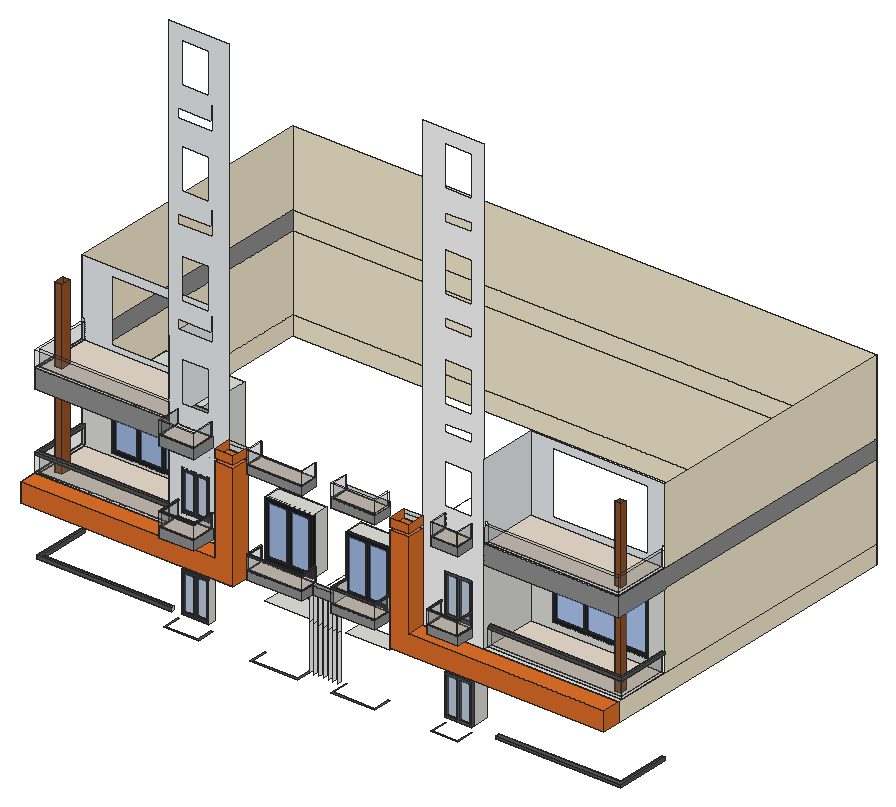
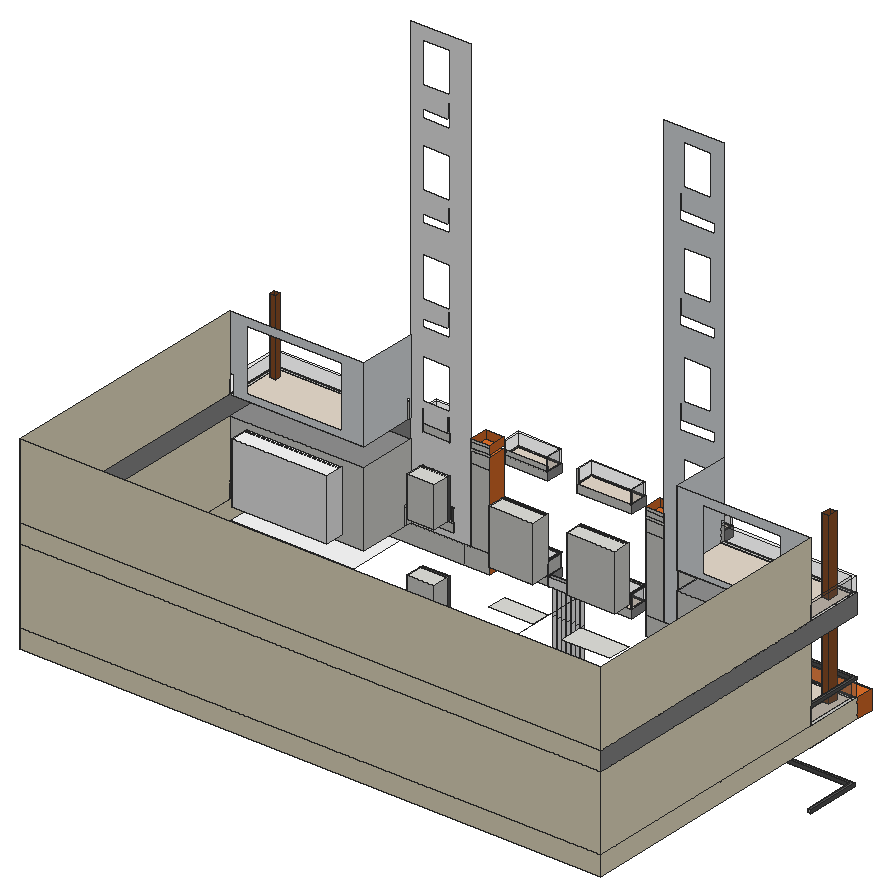
# SketchUp Ruby script. Lengths in inches.
U = 1.inch
M = Sketchup.active_model
def pt(a) = Geom::Point3d.new(a.map { |v| v * U })
def face(e, loops, mat)
  f = e.add_face(loops[0].map { |a| pt(a) })
  loops[1..].each { |l| e.add_face(l.map { |a| pt(a) }).erase! }
  f.material = f.back_material = mat if mat
  f
end
# faces: each face lists its corners as indices into pts; further lists are holes
def faces(e, pts, list, mat = nil) = list.each { |f| face(e, (f[0].is_a?(Array) ? f : [f]).map { |l| l.map { |i| pts[i] } }, mat) }
# xy, xz, yz: faces in a plane at the given z, y or x. An outline is a flat list of corners, or four numbers for a rectangle; further outlines are holes
def ring(l) = l.size == 4 ? [[l[0], l[1]], [l[2], l[1]], [l[2], l[3]], [l[0], l[3]]] : l.each_slice(2).to_a
def flat(e, list, mat, &to3) = list.each { |f| face(e, (f[0].is_a?(Array) ? f : [f]).map { |l| ring(l).map { |u, v| to3.(u, v) } }, mat) }
def xy(e, z, list, mat = nil) = flat(e, list, mat) { |x, y| [x, y, z] }
def xz(e, y, list, mat = nil) = flat(e, list, mat) { |x, z| [x, y, z] }
def yz(e, x, list, mat = nil) = flat(e, list, mat) { |y, z| [x, y, z] }
def lines(e, pts, list) = list.each { |a, b| e.add_line(pt(pts[a]), pt(pts[b])) }
# prism: a flat outline (further loops are holes) pulled along v
def prism(e, loops, v, mat = nil)
  f = face(e, loops, mat); d = Geom::Vector3d.new(v.map { |x| x * U })
  f.pushpull(f.normal.samedirection?(d) ? d.length : -d.length)
end
def box(e, o, s, mat = nil) = prism(e, [[o, [o[0] + s[0], o[1], o[2]], [o[0] + s[0], o[1] + s[1], o[2]], [o[0], o[1] + s[1], o[2]]]], [0, 0, s[2]], mat)
def at(x, y, z, deg = 0) = Geom::Transformation.translation(pt([x, y, z])) * Geom::Transformation.rotation(ORIGIN, Z_AXIS, deg.degrees)
def axes(o, x, y, z) = Geom::Transformation.new([*x, 0, *y, 0, *z, 0, *pt(o).to_a, 1])
def part(name) = M.definitions.add(name)
# library, detail: a bought-in or finely detailed component or shape, given as its bounding box
def library(name, o, s) = part(name).tap { |d| box(d.entities, o, s) }
def detail(e, o, s) = box(e.add_group.entities, o, s)
def put(e, d, t, mat = nil) = e.add_instance(d, t).tap { |i| i.material = mat if mat }
def group(e, t, mat = nil) = e.add_group.tap { |g| g.transformation = t; g.material = mat if mat }.entities
root = M.entities
M.materials.add("Generic").color = [146, 146, 146]
M.materials.add("Generic\#3").color = [226, 112, 41]
M.materials.add("Generic\#4").color = [237, 241, 244]
M.materials.add("Generic\#5").color = [249, 239, 211]
M.materials.add("Generic\#7").color = [232, 220, 205]
M.materials.add("[Color M00]").color = [255, 255, 255]
M.materials.add("[Color M06]").color = [86, 86, 86]
M.materials.add("[Color M07]").color = [58, 58, 58]
M.materials.add("[Color M08]").color = [30, 30, 30]
M.materials.add("[Translucent Glass Blue]").color = [98, 147, 234]
M.materials["[Translucent Glass Blue]"].alpha = 0.27
M.materials.add("[Translucent Glass Blue]1").color = [100, 149, 237]
M.materials["[Translucent Glass Blue]1"].alpha = 0.5
M.materials.add("[Translucent Glass Gray]").color = [119, 119, 119]
M.materials["[Translucent Glass Gray]"].alpha = 0.16
M.materials.add("[Wood Cherry Original]").color = [150, 85, 41]
M.materials.add("[Wood Cherry Original]1").color = [152, 86, 42]
c1 = part("Group\#1")
xy(c1.entities,0,[[0,0,60.75,6]],"[Color M07]")
xy(c1.entities,5.51,[[5.51,0,27.62,3],[33.13,0,55.24,3]],"[Color M07]")
xy(c1.entities,84.62,[[5.51,0,27.62,3],[33.13,0,55.24,3]])
xy(c1.entities,90.125,[[0,0,60.75,6]],"[Color M07]")
xz(c1.entities,0,[[[0,0,60.75,90.125],[5.51,5.51,27.62,84.62],[33.13,5.51,55.24,84.62]]],"[Color M07]")
xz(c1.entities,3,[[5.51,5.51,27.62,84.62],[33.13,5.51,55.24,84.62]],"[Translucent Glass Blue]")
xz(c1.entities,6,[[0,0,60.75,90.125]])
yz(c1.entities,0,[[0,0,6,90.125]],"[Color M07]")
yz(c1.entities,5.51,[[0,5.51,3,84.62]],"[Color M07]")
yz(c1.entities,27.62,[[0,5.51,3,84.62]],"[Color M07]")
yz(c1.entities,33.13,[[0,5.51,3,84.62]],"[Color M07]")
yz(c1.entities,55.24,[[0,5.51,3,84.62]],"[Color M07]")
yz(c1.entities,60.75,[[0,0,6,90.125]],"[Color M07]")
c2 = part("Group\#2")
xy(c2.entities,0,[[0,0,60.75,6]],"[Color M06]")
xy(c2.entities,4.875,[[4.875,0,27.9375,3],[32.8125,0,55.875,3]],"[Color M06]")
xy(c2.entities,85.25,[[4.875,0,27.9375,3],[32.8125,0,55.875,3]],"[Color M06]")
xy(c2.entities,90.125,[[0,0,60.75,6]],"[Color M06]")
xz(c2.entities,0,[[[0,0,60.75,90.125],[4.875,4.875,27.9375,85.25],[32.8125,4.875,55.875,85.25]]],"[Color M06]")
xz(c2.entities,3,[[4.875,4.875,27.9375,85.25],[32.8125,4.875,55.875,85.25]],"[Translucent Glass Blue]")
xz(c2.entities,6,[[0,0,60.75,90.125]])
yz(c2.entities,0,[[0,0,6,90.125]],"[Color M06]")
yz(c2.entities,4.875,[[0,4.875,3,85.25]],"[Color M06]")
yz(c2.entities,27.9375,[[0,4.875,3,85.25]],"[Color M06]")
yz(c2.entities,32.8125,[[0,4.875,3,85.25]],"[Color M06]")
yz(c2.entities,55.875,[[0,4.875,3,85.25]],"[Color M06]")
yz(c2.entities,60.75,[[0,0,6,90.125]],"[Color M06]")
c3 = part("Group\#10")
xy(c3.entities,0,[[0,0,98.1875,6]],"[Color M08]")
xy(c3.entities,5.79,[[5.79,0,46.2,3],[51.99,0,92.4,3]],"[Color M08]")
xy(c3.entities,117.02,[[5.79,0,46.2,3],[51.99,0,92.4,3]],"[Color M08]")
xy(c3.entities,122.8125,[[0,0,98.1875,6]],"[Color M08]")
xz(c3.entities,0,[[[0,0,98.1875,122.8125],[5.79,5.79,46.2,117.02],[51.99,5.79,92.4,117.02]]],"[Color M08]")
xz(c3.entities,3,[[5.79,5.79,46.2,117.02],[51.99,5.79,92.4,117.02]],"[Translucent Glass Blue]1")
xz(c3.entities,6,[[0,0,98.1875,122.8125]])
yz(c3.entities,0,[[0,0,6,122.8125]],"[Color M08]")
yz(c3.entities,5.79,[[0,5.79,3,117.02]],"[Color M08]")
yz(c3.entities,46.2,[[0,5.79,3,117.02]],"[Color M08]")
yz(c3.entities,51.99,[[0,5.79,3,117.02]],"[Color M08]")
yz(c3.entities,92.4,[[0,5.79,3,117.02]],"[Color M08]")
yz(c3.entities,98.1875,[[0,0,6,122.8125]],"[Color M08]")
c4 = part("Group\#11")
xy(c4.entities,0,[[0,0,175.8125,6]],"[Color M08]")
xy(c4.entities,7.33,[[7.33,0,56.16,3],[63.49,0,112.32,3],[119.65,0,168.48,3]],"[Color M08]")
xy(c4.entities,131.1,[[7.33,0,56.16,3],[63.49,0,112.32,3],[119.65,0,168.48,3]],"[Color M08]")
xy(c4.entities,138.4375,[[0,0,175.8125,6]],"[Color M08]")
xz(c4.entities,0,[[[0,0,175.8125,0,175.8125,131.1,168.48,131.1,168.48,7.33,119.65,7.33,119.65,131.1,175.8125,131.1,175.8125,138.4375,0,138.4375],[7.33,7.33,56.16,131.1],[63.49,7.33,112.32,131.1]]],"[Color M08]")
xz(c4.entities,3,[[7.33,7.33,56.16,131.1],[63.49,7.33,112.32,131.1],[119.65,7.33,168.48,131.1]],"[Translucent Glass Blue]1")
xz(c4.entities,6,[[0,0,175.8125,138.4375]])
yz(c4.entities,0,[[0,0,6,138.4375]],"[Color M08]")
yz(c4.entities,7.33,[[0,7.33,3,131.1]],"[Color M08]")
yz(c4.entities,56.16,[[0,7.33,3,131.1]],"[Color M08]")
yz(c4.entities,63.49,[[0,7.33,3,131.1]],"[Color M08]")
yz(c4.entities,112.32,[[0,7.33,3,131.1]],"[Color M08]")
yz(c4.entities,119.65,[[0,7.33,3,131.1]],"[Color M08]")
yz(c4.entities,168.48,[[0,7.33,3,131.1]],"[Color M08]")
yz(c4.entities,175.8125,[[0,0,6,138.4375]],"[Color M08]")
c5 = part("Group\#12")
xy(c5.entities,0,[[0,0,212.5625,7]],"[Color M08]")
xy(c5.entities,6.29,[[6.29,0,68.76,4],[75.05,0,137.52,4],[143.8,0,206.27,4]],"[Color M08]")
xy(c5.entities,131.21,[[6.29,0,68.76,4],[75.05,0,137.52,4],[143.8,0,206.27,4]],"[Color M08]")
xy(c5.entities,137.5,[[0,0,212.5625,7]],"[Color M08]")
xz(c5.entities,0,[[0,0,212.5625,6.29],[0,6.29,6.29,131.21],[68.76,6.29,75.05,131.21],[137.52,6.29,143.8,131.21],[206.27,6.29,212.5625,131.21],
  [0,131.21,212.5625,137.5]],"[Color M08]")
xz(c5.entities,4,[[6.29,6.29,68.76,131.21],[75.05,6.29,137.52,131.21],[143.8,6.29,206.27,131.21]],"[Translucent Glass Blue]1")
xz(c5.entities,7,[[0,0,212.5625,137.5]],"[Color M00]")
yz(c5.entities,0,[[0,0,7,137.5]],"[Color M08]")
yz(c5.entities,6.29,[[0,6.29,4,131.21]],"[Color M08]")
yz(c5.entities,68.76,[[0,6.29,4,131.21]],"[Color M08]")
yz(c5.entities,75.05,[[0,6.29,4,131.21]],"[Color M08]")
yz(c5.entities,137.52,[[0,6.29,4,131.21]],"[Color M08]")
yz(c5.entities,143.8,[[0,6.29,4,131.21]],"[Color M08]")
yz(c5.entities,206.27,[[0,6.29,4,131.21]],"[Color M08]")
yz(c5.entities,212.5625,[[0,0,7,137.5]],"[Color M08]")
xy(root,454.25,[[529.46,273.75,607.09,273.75,607.09,313.625,604.09,313.625,604.09,276.9375,532.46,276.9375,532.46,313.625,529.46,313.625]],"[Color M06]")
xy(root,454.5,[[722.84,273.75,830.21,273.75,830.21,313.625,827.21,313.625,827.21,276.75,725.84,276.75,725.84,313.625,722.84,313.625],[903.71,273.75,1001.9,273.75,1001.9,313.625,998.9,313.625,998.9,276.75,906.71,276.75,906.71,313.625,903.71,313.625],[1125.09,273.75,1185.84,273.75,1185.84,313.625,1182.84,313.625,1182.84,276.75,1128.09,276.75,1128.09,313.625,1125.09,313.625]],"[Color M06]")
xy(root,457.5,[[209.5,320.625,209.5,444.3125,216.5,444.3125,216.5,327.625,509.5,327.625,509.5,320.625]])
xy(root,457.5,[[1234.59,320.625,1234.59,329.25,1506,329.25,1506,444.3125,1513,444.3125,1513,320.625]],"[Color M00]")
xy(root,463.9375,[[1234.59,320.625,1513,320.625,1513,444.3125,1506,444.3125,1506,329.25,1234.59,329.25]],"[Color M06]")
xy(root,464.5,[[209.5,320.625,509.5,320.625,509.5,327.625,216.5,327.625,216.5,444.3125,209.5,444.3125]],"[Color M06]")
xy(root,465.5,[[537.9,313.625,598.65,331.25],[1125.09,313.625,1185.84,356.375]])
xy(root,555.62,[[537.9,313.625,598.65,331.25],[722.84,313.625,830.21,367.5],[903.71,313.625,1001.9,356.375],[1125.09,313.625,1185.84,356.375]])
xy(root,573.26,[[276.39,444.3125,452.2,595.9375]])
xy(root,577.32,[[1262.61,444.3125,1475.18,486.125]],"[Color M00]")
xy(root,589.5,[[[209.5,313.625,509.5,444.3125],[234.12,340.02,249.74,361.77]]])
xy(root,589.5,[[209.5,273.75,685.0625,313.625],[1034.5,273.75,1513,313.625]],"Generic\#3")
xy(root,589.5,[[[1234.59,313.625,1513,444.3125],[1483.76,340.63,1497.19,353.98]]],"[Color M00]")
xy(root,613.8125,[[714.9,273.75,714.9,313.625,830.21,313.625,830.21,305.3125,838.15,305.3125,838.15,273.75],[903.71,273.75,1001.9,313.625]],"Generic")
xy(root,613.8125,[[838.15,303.75,838.15,313.625,840.71,313.625,840.71,305.3125,848.65,305.3125,848.65,313.625,851.21,313.625,851.21,305.3125,859.15,305.3125,859.15,313.625,861.71,313.625,861.71,305.3125,869.65,305.3125,869.65,313.625,872.21,313.625,872.21,305.3125,880.15,305.3125,880.15,313.625,882.71,313.625,882.71,305.3125,890.65,305.3125,890.65,313.625,893.21,313.625,893.21,305.3125,901.15,305.3125,901.15,313.625,903.71,313.625,903.71,303.75],[830.21,305.3125,838.15,313.625],[840.71,305.3125,848.65,313.625],[851.21,305.3125,859.15,313.625],[861.71,305.3125,869.65,313.625],
  [872.21,305.3125,880.15,313.625],[882.71,305.3125,890.65,313.625],[893.21,305.3125,901.15,313.625]],"[Color M00]")
xy(root,632.25,[[714.9,273.75,838.15,276.75],[903.71,273.75,1001.9,276.75],[714.9,276.75,717.9,313.625],[835.15,276.75,838.15,313.625],[903.71,276.75,906.71,313.625],
  [998.9,276.75,1001.9,313.625],[209.5,313.625,509.5,320.625],[1213,313.625,1513,324.375],[209.5,320.625,216.5,444.3125],[1213,324.375,1213,331.375,1506,331.375,1506,444.3125,1513,444.3125,1513,324.375],
  [234.12,340.02,249.74,361.77],[1483.76,340.63,1497.19,353.98]])
xy(root,632.25,[[838.15,303.75,903.71,313.625]],"Generic")
xy(root,632.25,[[209.5,273.75,537.9,313.625],[537.9,273.75,643.375,313.625],[1076.1875,273.75,1513,313.625]],"Generic\#3")
xy(root,632.25,[[717.9,276.75,835.15,313.625],[906.71,276.75,998.9,313.625],[[216.5,320.625,509.5,444.3125],[234.12,340.02,249.74,361.77]],[[1213,331.375,1506,444.3125],[1483.76,340.63,1497.19,353.98]]],"Generic\#7")
xy(root,635.59,[[903.71,313.625,1001.9,356.375]])
xy(root,638.07,[[529.46,261.625,607.09,313.625]],"Generic")
xy(root,638.13,[[276.39,444.3125,452.2,595.9375]])
xy(root,638.46,[[722.84,313.625,830.21,353.375]])
xy(root,645.74,[[1116.15,273.75,1185.84,313.625]],"Generic")
xy(root,647.63,[[1262.61,444.3125,1475.18,486.125]],"[Color M00]")
xy(root,658.93,[[529.46,261.625,529.46,313.625,532.46,313.625,532.46,264.625,604.09,264.625,604.09,313.625,607.09,313.625,607.09,261.625]])
xy(root,658.93,[[532.46,264.625,604.09,313.625]],"Generic\#7")
xy(root,662.25,[[714.9,273.75,838.15,276.75],[903.71,273.75,1001.9,276.75],[714.9,276.75,717.9,313.625],[835.15,276.75,838.15,313.625],[903.71,276.75,906.71,313.625],
  [998.9,276.75,1001.9,313.625]])
xy(root,664.1,[[1116.15,273.75,1185.84,276.75],[1116.15,276.75,1119.71,313.625],[1182.84,276.75,1185.84,313.625]])
xy(root,664.1,[[1119.71,276.75,1182.84,313.625]],"Generic\#7")
xy(root,665.25,[[714.9,273.75,838.15,273.75,838.15,313.625,835.15,313.625,835.15,276.75,717.9,276.75,717.9,313.625,714.9,313.625],[903.71,273.75,1001.9,273.75,1001.9,313.625,998.9,313.625,998.9,276.75,906.71,276.75,906.71,313.625,903.71,313.625]],"[Color M06]")
xy(root,668.25,[[209.5,313.625,209.5,444.3125,216.5,444.3125,216.5,320.625,509.5,320.625,509.5,313.625],[1213,324.375,1213,331.375,1506,331.375,1506,444.3125,1513,444.3125,1513,324.375]])
xy(root,668.27,[[537.9,313.625,598.65,331.25],[1125.09,313.625,1185.84,356.375]])
xy(root,674.6875,[[1213,324.375,1513,324.375,1513,444.3125,1506,444.3125,1506,331.375,1213,331.375]],"[Color M06]")
xy(root,675.25,[[209.5,313.625,509.5,313.625,509.5,320.625,216.5,320.625,216.5,444.3125,209.5,444.3125]],"[Color M06]")
xy(root,688.93,[[529.46,261.625,529.46,313.625,532.46,313.625,532.46,264.625,604.09,264.625,604.09,313.625,607.09,313.625,607.09,261.625]])
xy(root,691.68,[[529.46,261.625,607.09,261.625,607.09,313.625,604.09,313.625,604.09,264.625,532.46,264.625,532.46,313.625,529.46,313.625]],"[Color M06]")
xy(root,694.1,[[1116.15,273.75,1185.84,276.75],[1116.15,276.75,1119.71,313.625],[1182.84,276.75,1185.84,313.625]])
xy(root,697.1,[[1116.15,273.75,1185.84,273.75,1185.84,313.625,1182.84,313.625,1182.84,276.75,1119.71,276.75,1119.71,313.625,1116.15,313.625]],"[Color M06]")
xy(root,758.4,[[537.9,313.625,598.65,331.25],[903.71,313.625,1001.9,356.375],[1125.09,313.625,1185.84,356.375]])
xy(root,764.34,[[722.84,313.625,830.21,353.375]])
xy(root,776.57,[[276.39,444.3125,452.2,595.9375]])
xy(root,785.13,[[1262.61,444.3125,1475.18,486.125]],"[Color M00]")
xy(root,800.25,[[[209.5,313.625,509.5,444.3125],[234.12,340.02,249.74,361.77]],[[1213,313.625,1513,444.3125],[1483.76,340.63,1497.19,353.98]]],"Generic")
xy(root,821.625,[[529.46,261.625,607.09,313.625]],"Generic")
xy(root,824.5625,[[714.9,273.75,838.15,313.625],[903.71,273.75,1001.9,313.625],[1125.09,273.75,1185.84,313.625]],"Generic")
xy(root,825.37,[[643.375,273.75,685.0625,313.625],[1034.5,273.75,1076.1875,313.625]],"Generic\#3")
xy(root,831.87,[[643.375,273.75,685.0625,313.625],[1034.5,273.75,1076.1875,313.625]],"Generic\#3")
xy(root,843,[[529.46,261.625,529.46,313.625,532.46,313.625,532.46,264.625,604.09,264.625,604.09,313.625,607.09,313.625,607.09,261.625],[714.9,273.75,838.15,276.75],[903.71,273.75,906.71,313.625],[906.71,273.75,1001.9,276.75],[1125.09,273.75,1185.84,276.75],
  [714.9,276.75,717.9,313.625],[835.15,276.75,838.15,313.625],[998.9,276.75,1001.9,313.625],[1125.09,276.75,1128.09,313.625],[1182.84,276.75,1185.84,313.625],
  [209.5,313.625,509.5,320.625],[537.9,313.625,598.65,318.125],[1213,313.625,1513,316.0625],[1213,316.0625,1213,323.0625,1506,323.0625,1506,444.3125,1513,444.3125,1513,316.0625],[209.5,320.625,216.5,444.3125],
  [234.12,340.02,249.74,361.77],[1483.76,340.63,1497.19,353.98]])
xy(root,843,[[532.46,264.625,604.09,313.625],[717.9,276.75,835.15,313.625],[906.71,276.75,998.9,313.625],[1128.09,276.75,1182.84,313.625],[[216.5,320.625,509.5,444.3125],[234.12,340.02,249.74,361.77]],
  [[1213,323.0625,1506,444.3125],[1483.76,340.63,1497.19,353.98]]],"Generic\#7")
xz(root,261.625,[[529.46,638.07,607.09,658.93],[529.46,821.625,607.09,843]],"Generic")
xz(root,261.625,[[529.46,688.93,607.09,691.68]],"[Color M06]")
xz(root,261.625,[[529.46,658.93,607.09,688.93],[529.46,843,607.09,873]],"[Translucent Glass Gray]")
xz(root,264.625,[[532.46,688.93,604.09,691.68]])
xz(root,264.625,[[532.46,658.93,604.09,688.93],[532.46,843,604.09,873]],"[Translucent Glass Gray]")
xz(root,273.75,[[714.9,613.8125,838.15,632.25],[903.71,613.8125,1001.9,632.25],[1116.15,645.74,1185.84,664.1],[714.9,824.5625,838.15,843],[903.71,824.5625,1001.9,843],
  [1125.09,824.5625,1185.84,843]],"Generic")
xz(root,273.75,[[209.5,589.5,685.0625,589.5,685.0625,825.37,643.375,825.37,643.375,632.25,209.5,632.25],[1034.5,589.5,1513,589.5,1513,632.25,1076.1875,632.25,1076.1875,825.37,1034.5,825.37],[643.375,831.87,685.0625,849.87],[1034.5,831.87,1076.1875,849.87]],"Generic\#3")
xz(root,273.75,[[714.9,662.25,838.15,665.25],[903.71,662.25,1001.9,665.25],[1116.15,694.1,1185.84,697.1]],"[Color M06]")
xz(root,273.75,[[714.9,632.25,838.15,662.25],[903.71,632.25,1001.9,662.25],[1116.15,664.1,1185.84,694.1],[714.9,843,838.15,873],[903.71,843,1001.9,873],
  [1125.09,843,1185.84,873]],"[Translucent Glass Gray]")
xz(root,276.75,[[717.9,662.25,835.15,665.25],[906.71,662.25,998.9,665.25],[1119.71,694.1,1182.84,697.1]])
xz(root,276.75,[[717.9,632.25,835.15,662.25],[906.71,632.25,998.9,662.25],[1119.71,664.1,1182.84,694.1],[717.9,843,835.15,873],[906.71,843,998.9,873],
  [1128.09,843,1182.84,873]],"[Translucent Glass Gray]")
xz(root,303.75,[[838.15,613.8125,903.71,632.25]],"Generic")
xz(root,313.625,[[209.5,589.5,629.5,632.25],[629.5,589.5,685.0625,632.25],[1034.5,589.5,1093,632.25],[1093,589.5,1513,632.25],[714.9,613.8125,838.15,632.25],
  [903.71,613.8125,1001.9,632.25],[643.375,632.25,685.0625,800.25],[714.9,632.25,717.9,662.25],[835.15,632.25,838.15,662.25],[903.71,632.25,906.71,635.59],
  [906.71,632.25,998.9,635.59],[998.9,632.25,1001.9,635.59],[1034.5,632.25,1076.1875,800.25],[903.71,635.59,906.71,662.25],[998.9,635.59,1001.9,662.25],
  [529.46,638.07,607.09,658.93],[1116.15,645.74,1185.84,664.1],[714.9,662.25,717.9,665.25],[835.15,662.25,838.15,665.25],[903.71,662.25,906.71,665.25],
  [998.9,662.25,1001.9,665.25],[1116.15,664.1,1119.71,668.27],[1182.84,664.1,1185.84,668.27],[1182.84,668.27,1185.84,694.1],[1116.15,694.1,1119.71,697.1],
  [1182.84,694.1,1185.84,697.1],[643.375,800.25,685.0625,825.37],[1034.5,800.25,1076.1875,825.37],[529.46,821.625,607.09,843],[714.9,824.5625,838.15,843],
  [903.71,824.5625,1001.9,843],[1125.09,824.5625,1185.84,843],[643.375,825.37,685.0625,831.87],[1034.5,825.37,1076.1875,831.87],[643.375,831.87,685.0625,843],
  [1034.5,831.87,1076.1875,843],[643.375,843,685.0625,849.87],[714.9,843,717.9,873],[835.15,843,838.15,873],[903.71,843,906.71,853.59],
  [906.71,843,998.9,853.59],[998.9,843,1001.9,853.59],[1034.5,843,1076.1875,849.87],[1125.09,843,1128.09,873],[1182.84,843,1185.84,873]])
xz(root,313.625,[[209.5,800.25,509.5,843],[1213,800.25,1513,843]],"Generic")
xz(root,313.625,[[[509.5,632.25,643.375,1643.25],[537.9,668.27,598.65,758.4],[537.9,1092.02,598.65,1182.15],[537.9,1523.77,598.65,1613.9],[537.9,1311.4,598.65,1401.52],[537.9,886.27,598.65,976.4],[529.46,1243.125,529.46,1297.25,532.46,1297.25,532.46,1264.5,604.09,1264.5,604.09,1297.25,607.09,1297.25,607.09,1243.125],[529.46,821.625,529.46,875.75,532.46,875.75,532.46,843,604.09,843,604.09,875.75,607.09,875.75,607.09,821.625],[529.46,1453.875,529.46,1508,532.46,1508,532.46,1475.25,604.09,1475.25,604.09,1508,607.09,1508,607.09,1453.875],[529.46,1032.375,529.46,1086.5,532.46,1086.5,532.46,1053.75,604.09,1053.75,604.09,1086.5,607.09,1086.5,607.09,1032.375],[529.46,638.07,529.46,691.68,532.46,691.68,532.46,658.93,604.09,658.93,604.09,691.68,607.09,691.68,607.09,638.07]]],"Generic\#4")
xz(root,313.625,[[838.15,613.8125,903.71,632.25],[[1076.1875,632.25,1213,1643.25],[1116.15,645.74,1185.84,645.74,1185.84,758.4,1125.09,758.4,1125.09,668.27,1182.84,668.27,1182.84,664.1,1119.71,664.1,1119.71,697.1,1116.15,697.1],[1125.09,887.24,1185.84,977.36],[1125.09,1092.02,1185.84,1182.15],[1125.09,1311.4,1185.84,1401.52],[1125.09,1523.77,1185.84,1613.9],[1125.09,1035.3125,1185.84,1035.3125,1185.84,1086.75,1182.84,1086.75,1182.84,1053.75,1128.09,1053.75,1128.09,1086.75,1125.09,1086.75],[1125.09,824.5625,1185.84,824.5625,1185.84,876,1182.84,876,1182.84,843,1128.09,843,1128.09,876,1125.09,876],[1125.09,1456.8125,1185.84,1456.8125,1185.84,1508.25,1182.84,1508.25,1182.84,1475.25,1128.09,1475.25,1128.09,1508.25,1125.09,1508.25],[1125.09,1246.0625,1185.84,1246.0625,1185.84,1297.5,1182.84,1297.5,1182.84,1264.5,1128.09,1264.5,1128.09,1297.5,1125.09,1297.5]]],"[Color M00]")
xz(root,313.625,[[209.5,668.25,509.5,675.25]],"[Color M06]")
xz(root,313.625,[[209.5,632.25,509.5,668.25],[1116.15,668.27,1119.71,694.1],[209.5,843,509.5,879]],"[Translucent Glass Gray]")
xz(root,316.0625,[[1213,843,1513,879]],"[Translucent Glass Gray]")
xz(root,318.125,[[537.9,800.25,598.65,843]])
xz(root,320.625,[[209.5,457.5,509.5,464.5],[1234.59,457.5,1513,463.9375],[216.5,668.25,509.5,675.25]],"[Color M06]")
xz(root,320.625,[[216.5,632.25,509.5,668.25],[216.5,843,509.5,879]],"[Translucent Glass Gray]")
xz(root,323.0625,[[1213,843,1506,879]],"[Translucent Glass Gray]")
xz(root,324.375,[[1213,668.25,1513,674.6875]],"[Color M06]")
xz(root,324.375,[[1213,632.25,1513,668.25]],"[Translucent Glass Gray]")
xz(root,327.625,[[216.5,457.5,509.5,464.5]],"[Color M06]")
xz(root,329.25,[[1234.59,457.5,1506,463.9375]],"[Color M06]")
xz(root,331.25,[[537.9,465.5,598.65,555.62],[537.9,668.27,598.65,758.4]])
xz(root,331.375,[[1213,668.25,1506,674.6875]],"[Color M06]")
xz(root,331.375,[[1213,632.25,1506,668.25]],"[Translucent Glass Gray]")
xz(root,340.02,[[234.12,632.25,249.74,800.25],[234.12,843,249.74,1011]],"[Wood Cherry Original]1")
xz(root,340.63,[[1483.76,632.25,1497.19,800.25],[1483.76,843,1497.19,1011]],"[Wood Cherry Original]")
xz(root,353.375,[[722.84,638.46,830.21,764.34]])
xz(root,353.98,[[1483.76,632.25,1497.19,800.25],[1483.76,843,1497.19,1011]],"[Wood Cherry Original]")
xz(root,356.375,[[1125.09,465.5,1185.84,555.62],[903.71,635.59,1001.9,758.4],[1125.09,668.27,1185.84,758.4]])
xz(root,361.77,[[234.12,632.25,249.74,800.25],[234.12,843,249.74,1011]],"[Wood Cherry Original]1")
xz(root,444.3125,[[209.5,457.5,216.5,464.5],[209.5,632.25,216.5,668.25],[[216.5,632.25,509.5,632.25,509.5,800.25,209.5,800.25,209.5,675.25,216.5,675.25],[276.39,638.13,452.2,776.57]],[[1213,632.25,1506,632.25,1506,674.6875,1513,674.6875,1513,800.25,1213,800.25],[1262.61,647.63,1475.18,785.13]],[209.5,668.25,216.5,675.25],
  [209.5,843,216.5,879]])
xz(root,444.3125,[[[216.5,843,509.5,843,509.5,1011,209.5,1011,209.5,886,216.5,886],[276.39,853.63,452.2,992.07]],[[1213,843,1506,843,1506,885.4375,1513,885.4375,1513,1011,1213,1011],[1262.61,856.82,1475.18,994.32]]],"Generic\#4")
xz(root,486.125,[[1262.61,647.63,1475.18,785.13]],"[Color M00]")
xz(root,595.9375,[[276.39,638.13,452.2,776.57]])
xz(root,1033.625,[[209.5,589.5,1513,632.25],[209.5,632.25,1513,800.25],[209.5,800.25,1513,843],[209.5,843,1513,1011]],"Generic\#5")
yz(root,209.5,[[313.625,800.25,1033.625,843]],"Generic")
yz(root,209.5,[[273.75,589.5,313.625,632.25]],"Generic\#3")
yz(root,209.5,[[313.625,589.5,1033.625,632.25],[444.3125,632.25,1033.625,800.25],[444.3125,843,1033.625,1011]],"Generic\#5")
yz(root,209.5,[[320.625,457.5,444.3125,464.5],[313.625,668.25,444.3125,675.25]],"[Color M06]")
yz(root,209.5,[[313.625,632.25,444.3125,668.25],[313.625,843,444.3125,879]],"[Translucent Glass Gray]")
yz(root,216.5,[[327.625,457.5,444.3125,464.5],[320.625,668.25,444.3125,675.25]],"[Color M06]")
yz(root,216.5,[[320.625,632.25,444.3125,668.25],[320.625,843,444.3125,879]],"[Translucent Glass Gray]")
yz(root,234.12,[[340.02,632.25,361.77,800.25],[340.02,843,361.77,1011]],"[Wood Cherry Original]1")
yz(root,249.74,[[340.02,632.25,361.77,800.25],[340.02,843,361.77,1011]],"[Wood Cherry Original]1")
yz(root,276.39,[[444.3125,638.13,595.9375,776.57]])
yz(root,452.2,[[444.3125,638.13,595.9375,776.57]])
yz(root,509.5,[[320.625,457.5,327.625,464.5],[313.625,632.25,320.625,668.25],[313.625,668.25,320.625,675.25],[313.625,843,320.625,879]])
yz(root,509.5,[[320.625,632.25,320.625,675.25,313.625,675.25,313.625,800.25,444.3125,800.25,444.3125,632.25],[320.625,843,320.625,886,313.625,886,313.625,1011,444.3125,1011,444.3125,843]],"Generic\#4")
yz(root,529.46,[[261.625,638.07,313.625,658.93],[261.625,821.625,313.625,843]],"Generic")
yz(root,529.46,[[261.625,688.93,313.625,691.68]],"[Color M06]")
yz(root,529.46,[[261.625,658.93,313.625,688.93],[261.625,843,313.625,873]],"[Translucent Glass Gray]")
yz(root,532.46,[[264.625,688.93,313.625,691.68]],"[Color M06]")
yz(root,532.46,[[264.625,658.93,313.625,688.93],[264.625,843,313.625,873]],"[Translucent Glass Gray]")
yz(root,537.9,[[313.625,465.5,331.25,555.62],[313.625,668.27,331.25,758.4]])
yz(root,598.65,[[313.625,465.5,331.25,555.62],[313.625,668.27,331.25,758.4]])
yz(root,604.09,[[264.625,688.93,313.625,691.68]],"[Color M06]")
yz(root,604.09,[[264.625,658.93,313.625,688.93],[264.625,843,313.625,873]],"[Translucent Glass Gray]")
yz(root,607.09,[[261.625,638.07,313.625,658.93],[261.625,821.625,313.625,843]],"Generic")
yz(root,607.09,[[261.625,688.93,313.625,691.68]],"[Color M06]")
yz(root,607.09,[[261.625,658.93,313.625,688.93],[261.625,843,313.625,873]],"[Translucent Glass Gray]")
yz(root,643.375,[[273.75,632.25,313.625,825.37],[273.75,831.87,313.625,849.87]],"Generic\#3")
yz(root,685.0625,[[273.75,589.5,313.625,825.37],[273.75,831.87,313.625,849.87]],"Generic\#3")
yz(root,714.9,[[273.75,662.25,313.625,665.25]])
yz(root,714.9,[[273.75,613.8125,313.625,632.25],[273.75,824.5625,313.625,843]],"Generic")
yz(root,714.9,[[273.75,632.25,313.625,662.25],[273.75,843,313.625,873]],"[Translucent Glass Gray]")
yz(root,717.9,[[276.75,662.25,313.625,665.25]],"[Color M06]")
yz(root,717.9,[[276.75,632.25,313.625,662.25],[276.75,843,313.625,873]],"[Translucent Glass Gray]")
yz(root,722.84,[[313.625,638.46,353.375,764.34]])
yz(root,830.21,[[313.625,638.46,353.375,764.34]])
yz(root,830.21,[[305.3125,454.5,313.625,555.62],[305.3125,555.62,313.625,613.8125]],"[Color M00]")
yz(root,835.15,[[276.75,662.25,313.625,665.25]],"[Color M06]")
yz(root,835.15,[[276.75,632.25,313.625,662.25],[276.75,843,313.625,873]],"[Translucent Glass Gray]")
yz(root,838.15,[[273.75,613.8125,303.75,632.25],[273.75,824.5625,313.625,843]],"Generic")
yz(root,838.15,[[303.75,613.8125,313.625,632.25]],"[Color M00]")
yz(root,838.15,[[273.75,662.25,313.625,665.25]],"[Color M06]")
yz(root,838.15,[[273.75,632.25,313.625,662.25],[273.75,843,313.625,873]],"[Translucent Glass Gray]")
yz(root,840.71,[[305.3125,454.5,313.625,555.62],[305.3125,555.62,313.625,613.8125]],"[Color M00]")
yz(root,851.21,[[305.3125,454.5,313.625,555.62],[305.3125,555.62,313.625,613.8125]],"[Color M00]")
yz(root,861.71,[[305.3125,454.5,313.625,555.62],[305.3125,555.62,313.625,613.8125]],"[Color M00]")
yz(root,872.21,[[305.3125,454.5,313.625,555.62],[305.3125,555.62,313.625,613.8125]],"[Color M00]")
yz(root,882.71,[[305.3125,454.5,313.625,555.62],[305.3125,555.62,313.625,613.8125]],"[Color M00]")
yz(root,893.21,[[305.3125,454.5,313.625,555.62],[305.3125,555.62,313.625,613.8125]],"[Color M00]")
yz(root,903.71,[[313.625,635.59,356.375,758.4]])
yz(root,903.71,[[273.75,613.8125,303.75,632.25],[273.75,824.5625,313.625,843]],"Generic")
yz(root,903.71,[[303.75,613.8125,313.625,632.25]],"[Color M00]")
yz(root,903.71,[[273.75,662.25,313.625,665.25]],"[Color M06]")
yz(root,903.71,[[273.75,632.25,313.625,662.25],[273.75,843,313.625,873]],"[Translucent Glass Gray]")
yz(root,906.71,[[276.75,632.25,313.625,662.25]])
yz(root,906.71,[[276.75,662.25,313.625,665.25]],"[Color M06]")
yz(root,906.71,[[276.75,843,313.625,873]],"[Translucent Glass Gray]")
yz(root,998.9,[[276.75,662.25,313.625,665.25]],"[Color M06]")
yz(root,998.9,[[276.75,632.25,313.625,662.25],[276.75,843,313.625,873]],"[Translucent Glass Gray]")
yz(root,1001.9,[[313.625,635.59,356.375,758.4]])
yz(root,1001.9,[[273.75,613.8125,313.625,632.25],[273.75,824.5625,313.625,843]],"Generic")
yz(root,1001.9,[[273.75,662.25,313.625,665.25]],"[Color M06]")
yz(root,1001.9,[[273.75,632.25,313.625,662.25],[273.75,843,313.625,873]],"[Translucent Glass Gray]")
yz(root,1034.5,[[273.75,589.5,313.625,825.37],[273.75,831.87,313.625,849.87]],"Generic\#3")
yz(root,1076.1875,[[273.75,632.25,313.625,825.37],[273.75,831.87,313.625,849.87]],"Generic\#3")
yz(root,1116.15,[[273.75,645.74,313.625,664.1]],"Generic")
yz(root,1116.15,[[273.75,694.1,313.625,697.1]],"[Color M06]")
yz(root,1116.15,[[273.75,664.1,313.625,694.1]],"[Translucent Glass Gray]")
yz(root,1119.71,[[276.75,694.1,313.625,697.1]],"[Color M06]")
yz(root,1119.71,[[276.75,664.1,313.625,694.1]],"[Translucent Glass Gray]")
yz(root,1125.09,[[313.625,465.5,356.375,555.62],[313.625,668.27,356.375,758.4]])
yz(root,1125.09,[[273.75,824.5625,313.625,843]],"Generic")
yz(root,1125.09,[[273.75,843,313.625,873]],"[Translucent Glass Gray]")
yz(root,1128.09,[[276.75,843,313.625,873]],"[Translucent Glass Gray]")
yz(root,1182.84,[[276.75,694.1,313.625,697.1]],"[Color M06]")
yz(root,1182.84,[[276.75,664.1,313.625,694.1],[276.75,843,313.625,873]],"[Translucent Glass Gray]")
yz(root,1185.84,[[313.625,465.5,356.375,555.62],[313.625,668.27,356.375,758.4]])
yz(root,1185.84,[[273.75,645.74,313.625,664.1],[273.75,824.5625,313.625,843]],"Generic")
yz(root,1185.84,[[273.75,694.1,313.625,697.1]],"[Color M06]")
yz(root,1185.84,[[273.75,664.1,313.625,694.1],[273.75,843,313.625,873]],"[Translucent Glass Gray]")
yz(root,1213,[[313.625,632.25,324.375,632.25,324.375,674.6875,331.375,674.6875,331.375,632.25,444.3125,632.25,444.3125,800.25,313.625,800.25],[324.375,632.25,331.375,668.25],[324.375,668.25,331.375,674.6875],[316.0625,843,323.0625,879]])
yz(root,1213,[[313.625,843,316.0625,843,316.0625,885.4375,323.0625,885.4375,323.0625,843,444.3125,843,444.3125,1011,313.625,1011]],"Generic\#4")
yz(root,1234.59,[[320.625,457.5,329.25,463.9375]],"[Color M00]")
yz(root,1262.61,[[444.3125,647.63,486.125,785.13]],"[Color M00]")
yz(root,1475.18,[[444.3125,647.63,486.125,785.13]],"[Color M00]")
yz(root,1483.76,[[340.63,632.25,353.98,800.25],[340.63,843,353.98,1011]],"[Wood Cherry Original]")
yz(root,1497.19,[[340.63,632.25,353.98,800.25],[340.63,843,353.98,1011]],"[Wood Cherry Original]")
yz(root,1506,[[329.25,457.5,444.3125,463.9375],[331.375,668.25,444.3125,674.6875]],"[Color M06]")
yz(root,1506,[[331.375,632.25,444.3125,668.25],[323.0625,843,444.3125,879]],"[Translucent Glass Gray]")
yz(root,1513,[[313.625,800.25,1033.625,843]],"Generic")
yz(root,1513,[[273.75,589.5,313.625,632.25]],"Generic\#3")
yz(root,1513,[[313.625,589.5,1033.625,632.25],[444.3125,632.25,1033.625,800.25],[444.3125,843,1033.625,1011]],"Generic\#5")
yz(root,1513,[[320.625,457.5,444.3125,463.9375],[324.375,668.25,444.3125,674.6875]],"[Color M06]")
yz(root,1513,[[324.375,632.25,444.3125,668.25],[316.0625,843,444.3125,879]],"[Translucent Glass Gray]")
p = [[598.65,313.625,800.25],[598.65,318.125,800.25],[537.9,313.625,800.25],[537.9,318.125,800.25],[838.15,313.625,613.8125],[838.15,803.75,613.8125]]
lines(root,p,[[0,1],[2,3],[4,5]])
put(root,c1,at(537.9,313.625,465.5))
put(root,c2,at(1125.09,313.625,465.5))
put(root,c3,at(903.71,313.625,635.59))
put(root,c4,at(276.39,444.3125,638.13))
g1 = group(root,at(722.84,313.625,638.46))
xy(g1,0,[[0,0,107.375,6]],"[Color M08]")
xy(g1,7.85,[[7.85,0,49.76,3],[57.61,0,99.52,3]],"[Color M08]")
xy(g1,118.02,[[7.85,0,49.76,3],[57.61,0,99.52,3]],"[Color M08]")
xy(g1,125.875,[[0,0,107.375,6]],"[Color M08]")
xz(g1,0,[[[0,0,107.375,125.875],[7.85,7.85,49.76,118.02],[57.61,7.85,99.52,118.02]]],"[Color M08]")
xz(g1,3,[[7.85,7.85,49.76,118.02],[57.61,7.85,99.52,118.02]],"[Translucent Glass Blue]1")
xz(g1,6,[[0,0,107.375,125.875]])
yz(g1,0,[[0,0,6,125.875]],"[Color M08]")
yz(g1,7.85,[[0,7.85,3,118.02]],"[Color M08]")
yz(g1,49.76,[[0,7.85,3,118.02]],"[Color M08]")
yz(g1,57.61,[[0,7.85,3,118.02]],"[Color M08]")
yz(g1,99.52,[[0,7.85,3,118.02]],"[Color M08]")
yz(g1,107.375,[[0,0,6,125.875]],"[Color M08]")
put(root,c5,at(1262.61,444.3125,647.63))
put(root,c2,at(1125.09,313.625,668.27))
put(root,c1,at(537.9,313.625,668.71))
